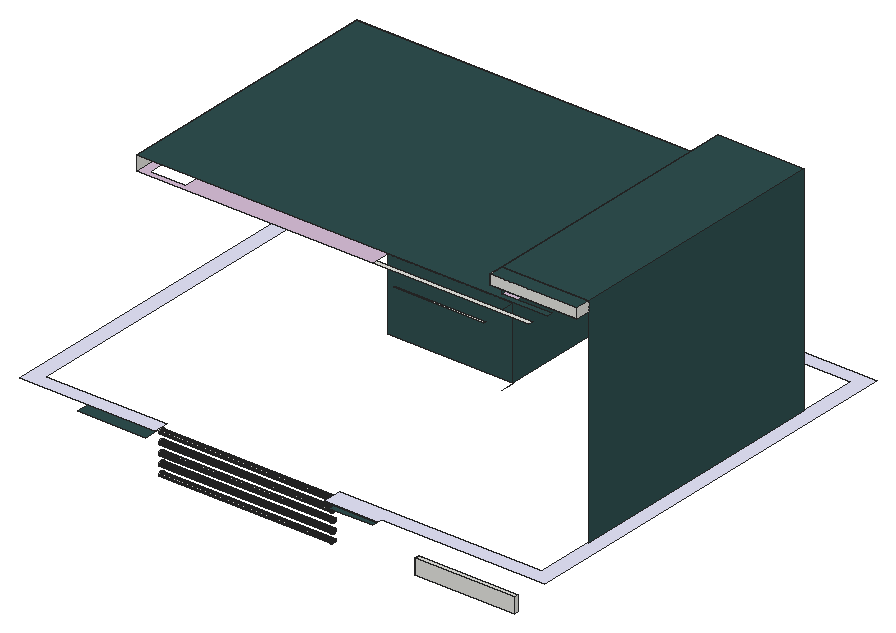
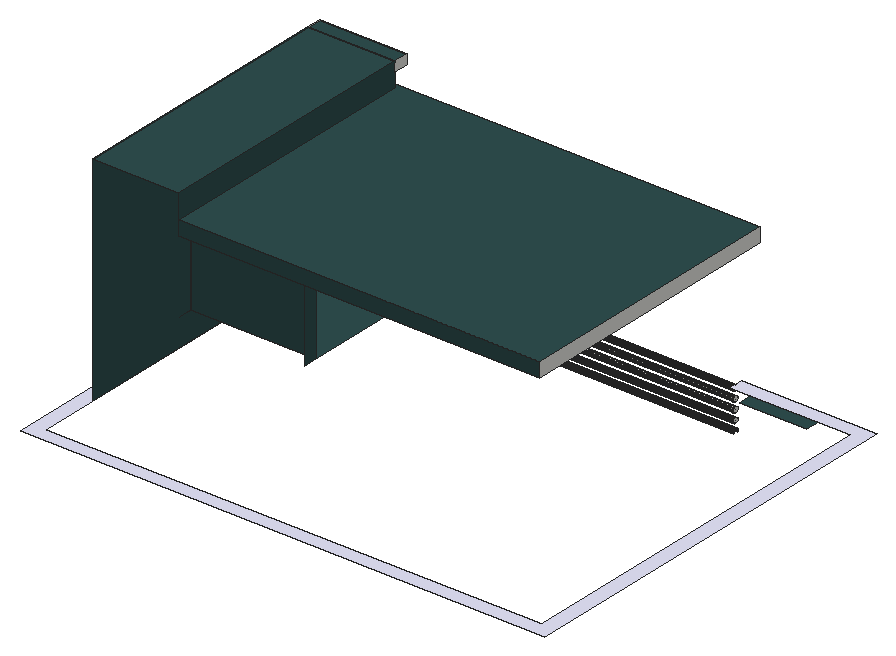
# SketchUp Ruby script. Lengths in inches.
U = 1.inch
M = Sketchup.active_model
def pt(a) = Geom::Point3d.new(a.map { |v| v * U })
def face(e, loops, mat)
  f = e.add_face(loops[0].map { |a| pt(a) })
  loops[1..].each { |l| e.add_face(l.map { |a| pt(a) }).erase! }
  f.material = f.back_material = mat if mat
  f
end
# faces: each face lists its corners as indices into pts; further lists are holes
def faces(e, pts, list, mat = nil) = list.each { |f| face(e, (f[0].is_a?(Array) ? f : [f]).map { |l| l.map { |i| pts[i] } }, mat) }
# xy, xz, yz: faces in a plane at the given z, y or x. An outline is a flat list of corners, or four numbers for a rectangle; further outlines are holes
def ring(l) = l.size == 4 ? [[l[0], l[1]], [l[2], l[1]], [l[2], l[3]], [l[0], l[3]]] : l.each_slice(2).to_a
def flat(e, list, mat, &to3) = list.each { |f| face(e, (f[0].is_a?(Array) ? f : [f]).map { |l| ring(l).map { |u, v| to3.(u, v) } }, mat) }
def xy(e, z, list, mat = nil) = flat(e, list, mat) { |x, y| [x, y, z] }
def xz(e, y, list, mat = nil) = flat(e, list, mat) { |x, z| [x, y, z] }
def yz(e, x, list, mat = nil) = flat(e, list, mat) { |y, z| [x, y, z] }
def lines(e, pts, list) = list.each { |a, b| e.add_line(pt(pts[a]), pt(pts[b])) }
# prism: a flat outline (further loops are holes) pulled along v
def prism(e, loops, v, mat = nil)
  f = face(e, loops, mat); d = Geom::Vector3d.new(v.map { |x| x * U })
  f.pushpull(f.normal.samedirection?(d) ? d.length : -d.length)
end
def box(e, o, s, mat = nil) = prism(e, [[o, [o[0] + s[0], o[1], o[2]], [o[0] + s[0], o[1] + s[1], o[2]], [o[0], o[1] + s[1], o[2]]]], [0, 0, s[2]], mat)
def at(x, y, z, deg = 0) = Geom::Transformation.translation(pt([x, y, z])) * Geom::Transformation.rotation(ORIGIN, Z_AXIS, deg.degrees)
def axes(o, x, y, z) = Geom::Transformation.new([*x, 0, *y, 0, *z, 0, *pt(o).to_a, 1])
def part(name) = M.definitions.add(name)
# library, detail: a bought-in or finely detailed component or shape, given as its bounding box
def library(name, o, s) = part(name).tap { |d| box(d.entities, o, s) }
def detail(e, o, s) = box(e.add_group.entities, o, s)
def put(e, d, t, mat = nil) = e.add_instance(d, t).tap { |i| i.material = mat if mat }
def group(e, t, mat = nil) = e.add_group.tap { |g| g.transformation = t; g.material = mat if mat }.entities
root = M.entities
M.materials.add("[0078_DarkSlateGray]").color = [47, 79, 79]
M.materials.add("[0116_Lavender]").color = [230, 230, 250]
M.materials.add("[0118_Thistle]").color = [216, 191, 216]
box(root,[607.99,0,329.13],[123.56,6,19.07])
xy(root,360,[[183,6,267,24]],"[0078_DarkSlateGray]")
xy(root,365.875,[[501.125,0,554.875,6]],"[0078_DarkSlateGray]")
xy(root,372,[[495,0,561,0,561,6,765,6,765,522,111,522,111,6,279,6,279,24,129,24,129,504,747,504,747,24,495,24]],"[0116_Lavender]")
xy(root,504,[[483,114,639,414]],"[0078_DarkSlateGray]")
xy(root,571.93,[[505.07,96,616.93,98]])
xy(root,594,[[483,90,677.8125,96]])
xy(root,594,[[[189,90,189,432,201,432,201,394.6875,245.25,394.6875,245.25,432,483,432,483,414,639,414,639,114,483,114,483,90],[201,96,245.25,133.3125],[306.12,131.99,309.21,132.55,312.04,133.88,314.44,135.9,316.22,138.47,317.29,141.42,317.55,144.54,317,147.62,315.67,150.46,313.65,152.85,311.08,154.64,308.13,155.7,305.01,155.97,301.93,155.42,299.09,154.08,296.7,152.0625,294.91,149.49,293.84,146.55,293.58,143.42,294.13,140.34,295.46,137.51,297.48,135.11,300.05,133.32,303,132.26],[415.43,131.99,418.52,132.55,421.35,133.88,423.75,135.9,425.54,138.47,426.6,141.42,426.86,144.54,426.3125,147.62,424.98,150.46,422.96,152.85,420.39,154.64,417.44,155.7,414.32,155.97,411.24,155.42,408.4,154.08,406.01,152.0625,404.22,149.49,403.16,146.55,402.89,143.42,403.44,140.34,404.78,137.51,406.8,135.11,409.37,133.32,412.3125,132.26],[415.43,355.81,418.52,356.36,421.35,357.69,423.75,359.71,425.54,362.28,426.6,365.23,426.86,368.35,426.3125,371.43,424.98,374.27,422.96,376.66,420.39,378.45,417.44,379.52,414.32,379.78,411.24,379.23,408.4,377.9,406.01,375.875,404.22,373.31,403.16,370.36,402.89,367.24,403.44,364.15,404.78,361.32,406.8,358.92,409.37,357.13,412.3125,356.07],[306.12,347.37,309.21,347.92,312.04,349.25,314.44,351.27,316.22,353.84,317.29,356.79,317.55,359.91,317,363,315.67,365.83,313.65,368.23,311.08,370.02,308.13,371.08,305.01,371.34,301.93,370.79,299.09,369.46,296.7,367.4375,294.91,364.87,293.84,361.92,293.58,358.8,294.13,355.72,295.46,352.88,297.48,350.49,300.05,348.7,303,347.63]]],"[0118_Thistle]")
xy(root,594.5,[[415.43,355.81,412.3125,356.07,409.37,357.13,406.8,358.92,404.78,361.32,403.44,364.15,402.89,367.24,403.16,370.36,404.22,373.31,406.01,375.875,408.4,377.9,411.24,379.23,414.32,379.78,417.44,379.52,420.39,378.45,422.96,376.66,424.98,374.27,426.3125,371.43,426.86,368.35,426.6,365.23,425.54,362.28,423.75,359.71,421.35,357.69,418.52,356.36]])
xy(root,594.9375,[[415.43,131.99,412.3125,132.26,409.37,133.32,406.8,135.11,404.78,137.51,403.44,140.34,402.89,143.42,403.16,146.55,404.22,149.49,406.01,152.0625,408.4,154.08,411.24,155.42,414.32,155.97,417.44,155.7,420.39,154.64,422.96,152.85,424.98,150.46,426.3125,147.62,426.86,144.54,426.6,141.42,425.54,138.47,423.75,135.9,421.35,133.88,418.52,132.55]])
xy(root,595.3125,[[306.12,347.37,303,347.63,300.05,348.7,297.48,350.49,295.46,352.88,294.13,355.72,293.58,358.8,293.84,361.92,294.91,364.87,296.7,367.4375,299.09,369.46,301.93,370.79,305.01,371.34,308.13,371.08,311.08,370.02,313.65,368.23,315.67,365.83,317,363,317.55,359.91,317.29,356.79,316.22,353.84,314.44,351.27,312.04,349.25,309.21,347.92]])
xy(root,595.4375,[[306.12,131.99,303,132.26,300.05,133.32,297.48,135.11,295.46,137.51,294.13,140.34,293.58,143.42,293.84,146.55,294.91,149.49,296.7,152.0625,299.09,154.08,301.93,155.42,305.01,155.97,308.13,155.7,311.08,154.64,313.65,152.85,315.67,150.46,317,147.62,317.55,144.54,317.29,141.42,316.22,138.47,314.44,135.9,312.04,133.88,309.21,132.55]])
xy(root,612,[[189,90,701.8125,90,701.8125,96,639,96,639,432,189,432]],"[0078_DarkSlateGray]")
xy(root,630,[[639,78,747,96]])
xy(root,642,[[639,78,747,96],[639,96,747,432]],"[0078_DarkSlateGray]")
xz(root,78,[[639,630,747,642]])
xz(root,96,[[639,630,747,642]])
xz(root,114,[[483,504,639,594]],"[0078_DarkSlateGray]")
xz(root,414,[[483,504,639,594]],"[0078_DarkSlateGray]")
xz(root,432,[[189,594,639,612]],"[0078_DarkSlateGray]")
yz(root,189,[[90,594,432,612]])
yz(root,279,[[15,328.75,14.22,328.85,13.5,329.15,12.88,329.625,12.4,330.25,12.1,330.97,12,331.75,12.1,332.52,12.4,333.25,12.88,333.87,13.5,334.34,14.22,334.64,15,334.75,15.78,334.64,16.5,334.34,17.12,333.87,17.6,333.25,17.9,332.52,18,331.75,17.9,330.97,17.6,330.25,17.12,329.625,16.5,329.15,15.78,328.85],[15,340.75,14.22,340.85,13.5,341.15,12.88,341.625,12.4,342.25,12.1,342.97,12,343.75,12.1,344.52,12.4,345.25,12.88,345.87,13.5,346.34,14.22,346.64,15,346.75,15.78,346.64,16.5,346.34,17.12,345.87,17.6,345.25,17.9,344.52,18,343.75,17.9,342.97,17.6,342.25,17.12,341.625,16.5,341.15,15.78,340.85],[15,352.75,14.22,352.85,13.5,353.15,12.88,353.625,12.4,354.25,12.1,354.97,12,355.75,12.1,356.52,12.4,357.25,12.88,357.87,13.5,358.34,14.22,358.64,15,358.75,15.78,358.64,16.5,358.34,17.12,357.87,17.6,357.25,17.9,356.52,18,355.75,17.9,354.97,17.6,354.25,17.12,353.625,16.5,353.15,15.78,352.85],[15,364.75,14.22,364.85,13.5,365.15,12.88,365.625,12.4,366.25,12.1,366.97,12,367.75,12.1,368.52,12.4,369.25,12.88,369.87,13.5,370.34,14.22,370.64,15,370.75,15.78,370.64,16.5,370.34,17.12,369.87,17.6,369.25,17.9,368.52,18,367.75,17.9,366.97,17.6,366.25,17.12,365.625,16.5,365.15,15.78,364.85]])
yz(root,483,[[414,504,432,594]],"[0078_DarkSlateGray]")
yz(root,639,[[78,630,96,642]])
yz(root,639,[[114,504,414,594],[96,612,432,642]],"[0078_DarkSlateGray]")
yz(root,747,[[78,630,96,642]])
yz(root,747,[[96,372,432,642]],"[0078_DarkSlateGray]")
p = [[279,12.1,318.97],[279,12.4,318.25],[495,12.4,318.25],[495,12.1,318.97],[279,17.6,318.25],[279,17.9,318.97],
  [495,17.9,318.97],[495,17.6,318.25],[279,12,319.75],[495,12,319.75],[279,18,319.75],[495,18,319.75],
  [279,12.1,320.52],[495,12.1,320.52],[279,17.9,320.52],[495,17.9,320.52],[279,12.4,321.25],[495,12.4,321.25],
  [279,17.6,321.25],[495,17.6,321.25],[279,12.88,321.87],[495,12.88,321.87],[279,17.12,321.87],[495,17.12,321.87],
  [279,13.5,322.34],[495,13.5,322.34],[279,16.5,322.34],[495,16.5,322.34],[279,14.22,322.64],[495,14.22,322.64],
  [279,15.78,322.64],[495,15.78,322.64],[279,15,322.75],[495,15,322.75],[279,14.22,328.85],[279,15,328.75],
  [495,15,328.75],[495,14.22,328.85],[279,15.78,328.85],[495,15.78,328.85],[279,13.5,329.15],[495,13.5,329.15],
  [279,16.5,329.15],[495,16.5,329.15],[279,12.88,329.625],[495,12.88,329.625],[279,17.12,329.625],[495,17.12,329.625],
  [279,12.4,330.25],[495,12.4,330.25],[279,17.6,330.25],[495,17.6,330.25],[279,12.1,330.97],[495,12.1,330.97],
  [279,17.9,330.97],[495,17.9,330.97],[279,12,331.75],[495,12,331.75],[279,18,331.75],[495,18,331.75],
  [279,12.1,332.52],[495,12.1,332.52],[279,17.9,332.52],[495,17.9,332.52],[279,12.4,333.25],[495,12.4,333.25],
  [279,17.6,333.25],[495,17.6,333.25],[279,12.88,333.87],[495,12.88,333.87],[279,17.12,333.87],[495,17.12,333.87],
  [279,13.5,334.34],[495,13.5,334.34],[279,16.5,334.34],[495,16.5,334.34],[279,14.22,334.64],[495,14.22,334.64],
  [279,15.78,334.64],[495,15.78,334.64],[279,15,334.75],[495,15,334.75],[279,14.22,340.85],[279,15,340.75],
  [495,15,340.75],[495,14.22,340.85],[279,15.78,340.85],[495,15.78,340.85],[279,13.5,341.15],[495,13.5,341.15],
  [279,16.5,341.15],[495,16.5,341.15],[279,12.88,341.625],[495,12.88,341.625],[279,17.12,341.625],[495,17.12,341.625],
  [279,12.4,342.25],[495,12.4,342.25],[279,17.6,342.25],[495,17.6,342.25],[279,12.1,342.97],[495,12.1,342.97],
  [279,17.9,342.97],[495,17.9,342.97],[279,12,343.75],[495,12,343.75],[279,18,343.75],[495,18,343.75],
  [279,12.1,344.52],[495,12.1,344.52],[279,17.9,344.52],[495,17.9,344.52],[279,12.4,345.25],[495,12.4,345.25],
  [279,17.6,345.25],[495,17.6,345.25],[279,12.88,345.87],[495,12.88,345.87],[279,17.12,345.87],[495,17.12,345.87],
  [279,13.5,346.34],[495,13.5,346.34],[279,16.5,346.34],[495,16.5,346.34],[279,14.22,346.64],[495,14.22,346.64],
  [279,15.78,346.64],[495,15.78,346.64],[279,15,346.75],[495,15,346.75],[279,14.22,352.85],[279,15,352.75],
  [495,15,352.75],[495,14.22,352.85],[279,15.78,352.85],[495,15.78,352.85],[279,13.5,353.15],[495,13.5,353.15],
  [279,16.5,353.15],[495,16.5,353.15],[279,12.88,353.625],[495,12.88,353.625],[279,17.12,353.625],[495,17.12,353.625],
  [279,12.4,354.25],[495,12.4,354.25],[279,17.6,354.25],[495,17.6,354.25],[279,12.1,354.97],[495,12.1,354.97],
  [279,17.9,354.97],[495,17.9,354.97],[279,12,355.75],[495,12,355.75],[279,18,355.75],[495,18,355.75],
  [279,12.1,356.52],[495,12.1,356.52],[279,17.9,356.52],[495,17.9,356.52],[279,12.4,357.25],[495,12.4,357.25],
  [279,17.6,357.25],[495,17.6,357.25],[279,12.88,357.87],[495,12.88,357.87],[279,17.12,357.87],[495,17.12,357.87],
  [279,13.5,358.34],[495,13.5,358.34],[279,16.5,358.34],[495,16.5,358.34],[279,14.22,358.64],[495,14.22,358.64],
  [279,15.78,358.64],[495,15.78,358.64],[279,15,358.75],[495,15,358.75],[279,14.22,364.85],[279,15,364.75],
  [495,15,364.75],[495,14.22,364.85],[279,15.78,364.85],[495,15.78,364.85],[279,13.5,365.15],[495,13.5,365.15],
  [279,16.5,365.15],[495,16.5,365.15],[279,12.88,365.625],[495,12.88,365.625],[279,17.12,365.625],[495,17.12,365.625],
  [279,12.4,366.25],[495,12.4,366.25],[279,17.6,366.25],[495,17.6,366.25],[279,12.1,366.97],[495,12.1,366.97],
  [279,17.9,366.97],[495,17.9,366.97],[279,12,367.75],[495,12,367.75],[279,18,367.75],[495,18,367.75],
  [279,12.1,368.52],[495,12.1,368.52],[279,17.9,368.52],[495,17.9,368.52],[279,12.4,369.25],[495,12.4,369.25],
  [279,17.6,369.25],[495,17.6,369.25],[279,12.88,369.87],[495,12.88,369.87],[279,17.12,369.87],[495,17.12,369.87],
  [279,13.5,370.34],[495,13.5,370.34],[279,16.5,370.34],[495,16.5,370.34],[279,14.22,370.64],[495,14.22,370.64],
  [279,15.78,370.64],[495,15.78,370.64],[279,15,370.75],[495,15,370.75],[306.12,131.99,594],[303,132.26,594],
  [303,132.26,595.4375],[306.12,131.99,595.4375],[309.21,132.55,594],[309.21,132.55,595.4375],[415.43,131.99,594],[412.3125,132.26,594],
  [412.3125,132.26,594.9375],[415.43,131.99,594.9375],[418.52,132.55,594],[418.52,132.55,594.9375],[300.05,133.32,594],[300.05,133.32,595.4375],
  [409.37,133.32,594],[409.37,133.32,594.9375],[312.04,133.88,594],[312.04,133.88,595.4375],[421.35,133.88,594],[421.35,133.88,594.9375],
  [297.48,135.11,594],[297.48,135.11,595.4375],[406.8,135.11,594],[406.8,135.11,594.9375],[314.44,135.9,594],[314.44,135.9,595.4375],
  [423.75,135.9,594],[423.75,135.9,594.9375],[295.46,137.51,594],[295.46,137.51,595.4375],[404.78,137.51,594],[404.78,137.51,594.9375],
  [316.22,138.47,594],[316.22,138.47,595.4375],[425.54,138.47,594],[425.54,138.47,594.9375],[294.13,140.34,594],[294.13,140.34,595.4375],
  [403.44,140.34,594],[403.44,140.34,594.9375],[317.29,141.42,594],[317.29,141.42,595.4375],[426.6,141.42,594],[426.6,141.42,594.9375],
  [293.58,143.42,594],[293.58,143.42,595.4375],[402.89,143.42,594],[402.89,143.42,594.9375],[317.55,144.54,594],[317.55,144.54,595.4375],
  [426.86,144.54,594],[426.86,144.54,594.9375],[293.84,146.55,594],[293.84,146.55,595.4375],[403.16,146.55,594],[403.16,146.55,594.9375],
  [317,147.62,594],[317,147.62,595.4375],[426.3125,147.62,594],[426.3125,147.62,594.9375],[294.91,149.49,594],[294.91,149.49,595.4375],
  [404.22,149.49,594],[404.22,149.49,594.9375],[315.67,150.46,594],[315.67,150.46,595.4375],[424.98,150.46,594],[424.98,150.46,594.9375],
  [296.7,152.0625,594],[296.7,152.0625,595.4375],[406.01,152.0625,594],[406.01,152.0625,594.9375],[313.65,152.85,594],[313.65,152.85,595.4375],
  [422.96,152.85,594],[422.96,152.85,594.9375],[299.09,154.08,594],[299.09,154.08,595.4375],[408.4,154.08,594],[408.4,154.08,594.9375],
  [311.08,154.64,594],[311.08,154.64,595.4375],[420.39,154.64,594],[420.39,154.64,594.9375],[301.93,155.42,594],[301.93,155.42,595.4375],
  [411.24,155.42,594],[411.24,155.42,594.9375],[308.13,155.7,594],[308.13,155.7,595.4375],[417.44,155.7,594],[417.44,155.7,594.9375],
  [305.01,155.97,594],[305.01,155.97,595.4375],[414.32,155.97,594],[414.32,155.97,594.9375],[306.12,347.37,594],[303,347.63,594],
  [303,347.63,595.3125],[306.12,347.37,595.3125],[309.21,347.92,594],[309.21,347.92,595.3125],[300.05,348.7,594],[300.05,348.7,595.3125],
  [312.04,349.25,594],[312.04,349.25,595.3125],[297.48,350.49,594],[297.48,350.49,595.3125],[314.44,351.27,594],[314.44,351.27,595.3125],
  [295.46,352.88,594],[295.46,352.88,595.3125],[316.22,353.84,594],[316.22,353.84,595.3125],[294.13,355.72,594],[294.13,355.72,595.3125],
  [317.29,356.79,594],[317.29,356.79,595.3125],[293.58,358.8,594],[293.58,358.8,595.3125],[415.43,355.81,594],[412.3125,356.07,594],
  [412.3125,356.07,594.5],[415.43,355.81,594.5],[418.52,356.36,594],[418.52,356.36,594.5],[409.37,357.13,594],[409.37,357.13,594.5],
  [421.35,357.69,594],[421.35,357.69,594.5],[317.55,359.91,594],[317.55,359.91,595.3125],[406.8,358.92,594],[406.8,358.92,594.5],
  [423.75,359.71,594],[423.75,359.71,594.5],[293.84,361.92,594],[293.84,361.92,595.3125],[404.78,361.32,594],[404.78,361.32,594.5],
  [425.54,362.28,594],[425.54,362.28,594.5],[317,363,594],[317,363,595.3125],[403.44,364.15,594],[403.44,364.15,594.5],
  [294.91,364.87,594],[294.91,364.87,595.3125],[426.6,365.23,594],[426.6,365.23,594.5],[315.67,365.83,594],[315.67,365.83,595.3125],
  [402.89,367.24,594],[402.89,367.24,594.5],[296.7,367.4375,594],[296.7,367.4375,595.3125],[426.86,368.35,594],[426.86,368.35,594.5],
  [313.65,368.23,594],[313.65,368.23,595.3125],[403.16,370.36,594],[403.16,370.36,594.5],[299.09,369.46,594],[299.09,369.46,595.3125],
  [311.08,370.02,594],[311.08,370.02,595.3125],[426.3125,371.43,594],[426.3125,371.43,594.5],[301.93,370.79,594],[301.93,370.79,595.3125],
  [308.13,371.08,594],[308.13,371.08,595.3125],[404.22,373.31,594],[404.22,373.31,594.5],[305.01,371.34,594],[305.01,371.34,595.3125],
  [424.98,374.27,594],[424.98,374.27,594.5],[406.01,375.875,594],[406.01,375.875,594.5],[422.96,376.66,594],[422.96,376.66,594.5],
  [408.4,377.9,594],[408.4,377.9,594.5],[420.39,378.45,594],[420.39,378.45,594.5],[411.24,379.23,594],[411.24,379.23,594.5],
  [417.44,379.52,594],[417.44,379.52,594.5],[414.32,379.78,594],[414.32,379.78,594.5],[639,96,594],[639,114,594],
  [639,114,504],[639,96,504],[639,414,504],[639,432,504],[639,414,594],[639,432,594],
  [279,15,319.75],[495,15,319.75],[279,15,331.75],[495,15,331.75],[279,15,343.75],[495,15,343.75],
  [279,15,355.75],[495,15,355.75],[279,15,367.75],[495,15,367.75]]
faces(root,p,[[0,1,2,3],[4,5,6,7],[8,0,3,9],[5,10,11,6],[12,8,9,13],[10,14,15,11],[16,12,13,17],[14,18,19,15],
  [20,16,17,21],[18,22,23,19],[24,20,21,25],[22,26,27,23],[28,24,25,29],[26,30,31,27],[32,28,29,33],[30,32,33,31],
  [34,35,36,37],[35,38,39,36],[40,34,37,41],[38,42,43,39],[44,40,41,45],[42,46,47,43],[48,44,45,49],[46,50,51,47],
  [52,48,49,53],[50,54,55,51],[56,52,53,57],[54,58,59,55],[60,56,57,61],[58,62,63,59],[64,60,61,65],[62,66,67,63],
  [68,64,65,69],[66,70,71,67],[72,68,69,73],[70,74,75,71],[76,72,73,77],[74,78,79,75],[80,76,77,81],[78,80,81,79],
  [82,83,84,85],[83,86,87,84],[88,82,85,89],[86,90,91,87],[92,88,89,93],[90,94,95,91],[96,92,93,97],[94,98,99,95],
  [100,96,97,101],[98,102,103,99],[104,100,101,105],[102,106,107,103],[108,104,105,109],[106,110,111,107],[112,108,109,113],[110,114,115,111],
  [116,112,113,117],[114,118,119,115],[120,116,117,121],[118,122,123,119],[124,120,121,125],[122,126,127,123],[128,124,125,129],[126,128,129,127],
  [130,131,132,133],[131,134,135,132],[136,130,133,137],[134,138,139,135],[140,136,137,141],[138,142,143,139],[144,140,141,145],[142,146,147,143],
  [148,144,145,149],[146,150,151,147],[152,148,149,153],[150,154,155,151],[156,152,153,157],[154,158,159,155],[160,156,157,161],[158,162,163,159],
  [164,160,161,165],[162,166,167,163],[168,164,165,169],[166,170,171,167],[172,168,169,173],[170,174,175,171],[176,172,173,177],[174,176,177,175],
  [178,179,180,181],[179,182,183,180],[184,178,181,185],[182,186,187,183],[188,184,185,189],[186,190,191,187],[192,188,189,193],[190,194,195,191],
  [196,192,193,197],[194,198,199,195],[200,196,197,201],[198,202,203,199],[204,200,201,205],[202,206,207,203],[208,204,205,209],[206,210,211,207],
  [212,208,209,213],[210,214,215,211],[216,212,213,217],[214,218,219,215],[220,216,217,221],[218,222,223,219],[224,220,221,225],[222,224,225,223],
  [226,227,228,229],[230,226,229,231],[232,233,234,235],[236,232,235,237],[227,238,239,228],[233,240,241,234],[242,230,231,243],[244,236,237,245],
  [238,246,247,239],[240,248,249,241],[250,242,243,251],[252,244,245,253],[246,254,255,247],[248,256,257,249],[258,250,251,259],[260,252,253,261],
  [254,262,263,255],[256,264,265,257],[266,258,259,267],[268,260,261,269],[262,270,271,263],[264,272,273,265],[274,266,267,275],[276,268,269,277],
  [270,278,279,271],[272,280,281,273],[282,274,275,283],[284,276,277,285],[278,286,287,279],[280,288,289,281],[290,282,283,291],[292,284,285,293],
  [286,294,295,287],[288,296,297,289],[298,290,291,299],[300,292,293,301],[294,302,303,295],[296,304,305,297],[306,298,299,307],[308,300,301,309],
  [302,310,311,303],[304,312,313,305],[314,306,307,315],[316,308,309,317],[310,318,319,311],[312,320,321,313],[318,314,315,319],[320,316,317,321],
  [322,323,324,325],[326,322,325,327],[323,328,329,324],[330,326,327,331],[328,332,333,329],[334,330,331,335],[332,336,337,333],[338,334,335,339],
  [336,340,341,337],[342,338,339,343],[340,344,345,341],[346,347,348,349],[350,346,349,351],[347,352,353,348],[354,350,351,355],[356,342,343,357],
  [352,358,359,353],[360,354,355,361],[344,362,363,345],[358,364,365,359],[366,360,361,367],[368,356,357,369],[364,370,371,365],[362,372,373,363],
  [374,366,367,375],[376,368,369,377],[370,378,379,371],[372,380,381,373],[382,374,375,383],[384,376,377,385],[378,386,387,379],[380,388,389,381],
  [390,384,385,391],[392,382,383,393],[388,394,395,389],[396,390,391,397],[386,398,399,387],[394,400,401,395],[400,396,397,401],[402,392,393,403],
  [398,404,405,399],[406,402,403,407],[404,408,409,405],[410,406,407,411],[408,412,413,409],[414,410,411,415],[412,416,417,413],[416,414,415,417]])
lines(root,p,[[418,419],[420,421],[422,423],[424,425],[426,427],[428,429],[430,431],[432,433],[434,435]])
